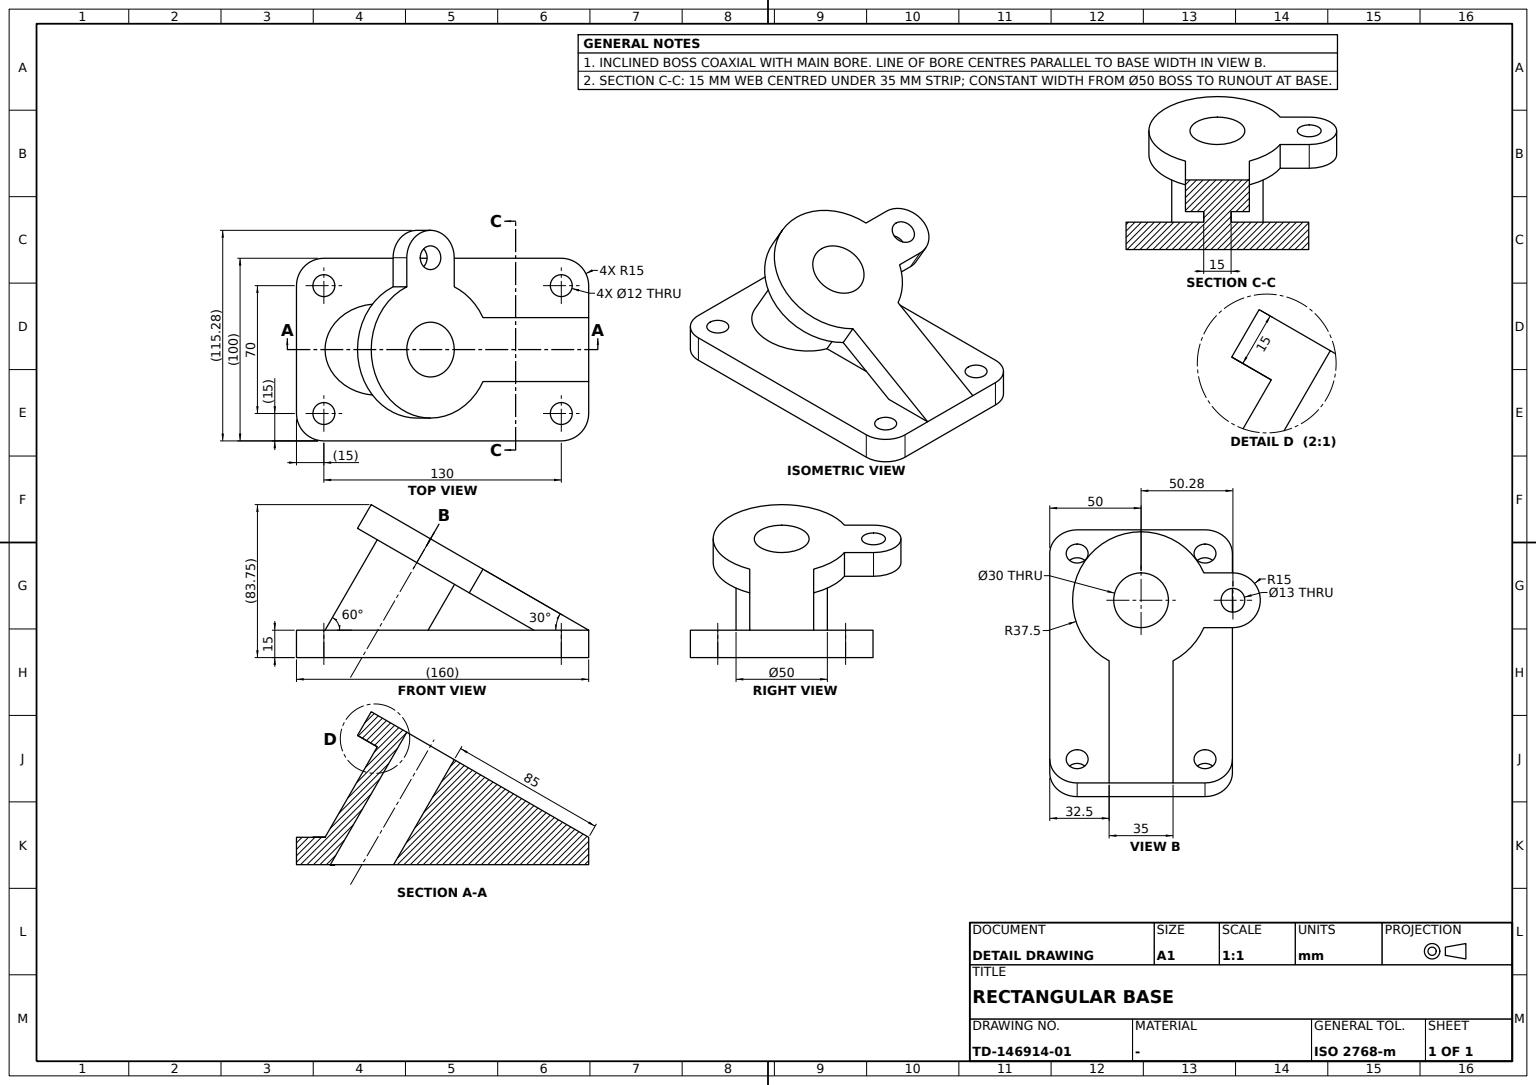
ISO-10303-21;
HEADER;
FILE_DESCRIPTION((''),'2;1');
FILE_NAME('','',(''),(''),'','','');
FILE_SCHEMA(('AUTOMOTIVE_DESIGN'));
ENDSEC;
DATA;
#1=APPLICATION_CONTEXT('');
#2=PRODUCT_CONTEXT('',#1,'mechanical');
#3=PRODUCT('','','',(#2));
#4=PRODUCT_DEFINITION_FORMATION('','',#3);
#5=PRODUCT_DEFINITION_CONTEXT('',#1,'design');
#6=PRODUCT_DEFINITION('','',#4,#5);
#7=PRODUCT_DEFINITION_SHAPE('','',#6);
#8=(LENGTH_UNIT()NAMED_UNIT(*)SI_UNIT(.MILLI.,.METRE.));
#9=(NAMED_UNIT(*)PLANE_ANGLE_UNIT()SI_UNIT($,.RADIAN.));
#10=(NAMED_UNIT(*)SI_UNIT($,.STERADIAN.)SOLID_ANGLE_UNIT());
#11=UNCERTAINTY_MEASURE_WITH_UNIT(LENGTH_MEASURE(0.005),#8,'distance_accuracy_value','');
#12=(GEOMETRIC_REPRESENTATION_CONTEXT(3)GLOBAL_UNCERTAINTY_ASSIGNED_CONTEXT((#11))GLOBAL_UNIT_ASSIGNED_CONTEXT((#8,#9,#10))REPRESENTATION_CONTEXT('',''));
#13=CARTESIAN_POINT('',(-59.,-35.,15.));
#14=VERTEX_POINT('',#13);
#15=CARTESIAN_POINT('',(-71.,-35.,15.));
#16=VERTEX_POINT('',#15);
#17=CARTESIAN_POINT('',(-65.,-35.,15.));
#18=DIRECTION('',(0.,0.,1.));
#19=DIRECTION('',(1.,0.,0.));
#20=AXIS2_PLACEMENT_3D('',#17,#18,#19);
#21=CIRCLE('',#20,6.);
#22=EDGE_CURVE('',#14,#16,#21,.T.);
#23=ORIENTED_EDGE('',*,*,#22,.F.);
#24=EDGE_CURVE('',#16,#14,#21,.T.);
#25=ORIENTED_EDGE('',*,*,#24,.F.);
#26=EDGE_LOOP('',(#23,#25));
#27=FACE_BOUND('',#26,.T.);
#28=CARTESIAN_POINT('',(59.,-35.,15.));
#29=VERTEX_POINT('',#28);
#30=CARTESIAN_POINT('',(71.,-35.,15.));
#31=VERTEX_POINT('',#30);
#32=CARTESIAN_POINT('',(65.,-35.,15.));
#33=AXIS2_PLACEMENT_3D('',#32,#18,#19);
#34=CIRCLE('',#33,6.);
#35=EDGE_CURVE('',#29,#31,#34,.T.);
#36=ORIENTED_EDGE('',*,*,#35,.F.);
#37=EDGE_CURVE('',#31,#29,#34,.T.);
#38=ORIENTED_EDGE('',*,*,#37,.F.);
#39=EDGE_LOOP('',(#36,#38));
#40=FACE_BOUND('',#39,.T.);
#41=CARTESIAN_POINT('',(-71.,35.,15.));
#42=VERTEX_POINT('',#41);
#43=CARTESIAN_POINT('',(-59.,35.,15.));
#44=VERTEX_POINT('',#43);
#45=CARTESIAN_POINT('',(-65.,35.,15.));
#46=AXIS2_PLACEMENT_3D('',#45,#18,#19);
#47=CIRCLE('',#46,6.);
#48=EDGE_CURVE('',#42,#44,#47,.T.);
#49=ORIENTED_EDGE('',*,*,#48,.F.);
#50=EDGE_CURVE('',#44,#42,#47,.T.);
#51=ORIENTED_EDGE('',*,*,#50,.F.);
#52=EDGE_LOOP('',(#49,#51));
#53=FACE_BOUND('',#52,.T.);
#54=CARTESIAN_POINT('',(71.,35.,15.));
#55=VERTEX_POINT('',#54);
#56=CARTESIAN_POINT('',(59.,35.,15.));
#57=VERTEX_POINT('',#56);
#58=CARTESIAN_POINT('',(65.,35.,15.));
#59=AXIS2_PLACEMENT_3D('',#58,#18,#19);
#60=CIRCLE('',#59,6.);
#61=EDGE_CURVE('',#55,#57,#60,.T.);
#62=ORIENTED_EDGE('',*,*,#61,.F.);
#63=EDGE_CURVE('',#57,#55,#60,.T.);
#64=ORIENTED_EDGE('',*,*,#63,.F.);
#65=EDGE_LOOP('',(#62,#64));
#66=FACE_BOUND('',#65,.T.);
#67=CARTESIAN_POINT('',(80.,17.5,15.));
#68=VERTEX_POINT('',#67);
#69=CARTESIAN_POINT('',(80.,35.,15.));
#70=VERTEX_POINT('',#69);
#71=CARTESIAN_POINT('',(80.,-35.,15.));
#72=DIRECTION('',(0.,1.,0.));
#73=VECTOR('',#72,1000.);
#74=LINE('',#71,#73);
#75=EDGE_CURVE('',#68,#70,#74,.T.);
#76=ORIENTED_EDGE('',*,*,#75,.T.);
#77=CARTESIAN_POINT('',(65.,50.,15.));
#78=VERTEX_POINT('',#77);
#79=CIRCLE('',#59,15.);
#80=EDGE_CURVE('',#70,#78,#79,.T.);
#81=ORIENTED_EDGE('',*,*,#80,.T.);
#82=CARTESIAN_POINT('',(-65.,50.,15.));
#83=VERTEX_POINT('',#82);
#84=DIRECTION('',(-1.,0.,0.));
#85=VECTOR('',#84,1000.);
#86=LINE('',#77,#85);
#87=EDGE_CURVE('',#78,#83,#86,.T.);
#88=ORIENTED_EDGE('',*,*,#87,.T.);
#89=CARTESIAN_POINT('',(-80.,35.,15.));
#90=VERTEX_POINT('',#89);
#91=CIRCLE('',#46,15.);
#92=EDGE_CURVE('',#83,#90,#91,.T.);
#93=ORIENTED_EDGE('',*,*,#92,.T.);
#94=CARTESIAN_POINT('',(-80.,-35.,15.));
#95=VERTEX_POINT('',#94);
#96=DIRECTION('',(0.,-1.,0.));
#97=VECTOR('',#96,1000.);
#98=LINE('',#89,#97);
#99=EDGE_CURVE('',#90,#95,#98,.T.);
#100=ORIENTED_EDGE('',*,*,#99,.T.);
#101=CARTESIAN_POINT('',(-65.,-50.,15.));
#102=VERTEX_POINT('',#101);
#103=CIRCLE('',#20,15.);
#104=EDGE_CURVE('',#95,#102,#103,.T.);
#105=ORIENTED_EDGE('',*,*,#104,.T.);
#106=CARTESIAN_POINT('',(65.,-50.,15.));
#107=VERTEX_POINT('',#106);
#108=VECTOR('',#19,1000.);
#109=LINE('',#101,#108);
#110=EDGE_CURVE('',#102,#107,#109,.T.);
#111=ORIENTED_EDGE('',*,*,#110,.T.);
#112=VERTEX_POINT('',#71);
#113=CIRCLE('',#33,15.);
#114=EDGE_CURVE('',#107,#112,#113,.T.);
#115=ORIENTED_EDGE('',*,*,#114,.T.);
#116=CARTESIAN_POINT('',(80.,-17.5,15.));
#117=VERTEX_POINT('',#116);
#118=EDGE_CURVE('',#112,#117,#74,.T.);
#119=ORIENTED_EDGE('',*,*,#118,.T.);
#120=CARTESIAN_POINT('',(50.,-17.5,15.));
#121=VERTEX_POINT('',#120);
#122=CARTESIAN_POINT('',(22.120273,-17.5,15.));
#123=LINE('',#122,#108);
#124=EDGE_CURVE('',#121,#117,#123,.T.);
#125=ORIENTED_EDGE('',*,*,#124,.F.);
#126=CARTESIAN_POINT('',(50.,-7.5,15.));
#127=VERTEX_POINT('',#126);
#128=CARTESIAN_POINT('',(50.,0.,15.));
#129=LINE('',#128,#97);
#130=EDGE_CURVE('',#127,#121,#129,.T.);
#131=ORIENTED_EDGE('',*,*,#130,.F.);
#132=CARTESIAN_POINT('',(-7.932201,-7.5,15.));
#133=VERTEX_POINT('',#132);
#134=CARTESIAN_POINT('',(-65.,-7.5,15.));
#135=LINE('',#134,#85);
#136=EDGE_CURVE('',#127,#133,#135,.T.);
#137=ORIENTED_EDGE('',*,*,#136,.T.);
#138=CARTESIAN_POINT('',(-64.337567,0.,15.));
#139=VERTEX_POINT('',#138);
#140=CARTESIAN_POINT('',(-64.337567,-37.913542,15.));
#141=CARTESIAN_POINT('',(-21.065837,-43.667214,15.));
#142=(BOUNDED_CURVE()B_SPLINE_CURVE(3,(#138,#140,#141,#132),.UNSPECIFIED.,.F.,.F.)B_SPLINE_CURVE_WITH_KNOTS((4,4),(0.,2.8369),.UNSPECIFIED.)CURVE()GEOMETRIC_REPRESENTATION_ITEM()RATIONAL_B_SPLINE_CURVE((1.,0.434505133,0.434505133,1.))REPRESENTATION_ITEM(''));
#143=EDGE_CURVE('',#139,#133,#142,.T.);
#144=ORIENTED_EDGE('',*,*,#143,.F.);
#145=CARTESIAN_POINT('',(-7.932201,7.5,15.));
#146=VERTEX_POINT('',#145);
#147=CARTESIAN_POINT('',(-21.065837,43.667214,15.));
#148=CARTESIAN_POINT('',(-64.337567,37.913542,15.));
#149=(BOUNDED_CURVE()B_SPLINE_CURVE(3,(#145,#147,#148,#138),.UNSPECIFIED.,.F.,.F.)B_SPLINE_CURVE_WITH_KNOTS((4,4),(3.446285308,6.283185307),.UNSPECIFIED.)CURVE()GEOMETRIC_REPRESENTATION_ITEM()RATIONAL_B_SPLINE_CURVE((1.,0.434505133,0.434505133,1.))REPRESENTATION_ITEM(''));
#150=EDGE_CURVE('',#146,#139,#149,.T.);
#151=ORIENTED_EDGE('',*,*,#150,.F.);
#152=CARTESIAN_POINT('',(50.,7.5,15.));
#153=VERTEX_POINT('',#152);
#154=CARTESIAN_POINT('',(-65.,7.5,15.));
#155=LINE('',#154,#108);
#156=EDGE_CURVE('',#146,#153,#155,.T.);
#157=ORIENTED_EDGE('',*,*,#156,.T.);
#158=CARTESIAN_POINT('',(50.,17.5,15.));
#159=VERTEX_POINT('',#158);
#160=EDGE_CURVE('',#159,#153,#129,.T.);
#161=ORIENTED_EDGE('',*,*,#160,.F.);
#162=LINE('',#67,#85);
#163=EDGE_CURVE('',#68,#159,#162,.T.);
#164=ORIENTED_EDGE('',*,*,#163,.F.);
#165=EDGE_LOOP('',(#76,#81,#88,#93,#100,#105,#111,#115,#119,#125,#131,#137,#144,#151,#157,#161,#164));
#166=FACE_BOUND('',#165,.T.);
#167=PLANE('',#20);
#168=ADVANCED_FACE('',(#27,#40,#53,#66,#166),#167,.T.);
#169=CARTESIAN_POINT('',(-35.753175,0.,64.509619));
#170=VERTEX_POINT('',#169);
#171=CARTESIAN_POINT('',(6.550849,7.5,40.085379));
#172=VERTEX_POINT('',#171);
#173=CARTESIAN_POINT('',(-14.10254,0.,52.009619));
#174=DIRECTION('',(-0.5,0.,-0.866025404));
#175=DIRECTION('',(0.866025404,0.,-0.5));
#176=AXIS2_PLACEMENT_3D('',#173,#174,#175);
#177=CIRCLE('',#176,25.);
#178=EDGE_CURVE('',#170,#172,#177,.T.);
#179=ORIENTED_EDGE('',*,*,#178,.F.);
#180=CARTESIAN_POINT('',(6.550849,-7.5,40.085379));
#181=VERTEX_POINT('',#180);
#182=EDGE_CURVE('',#181,#170,#177,.T.);
#183=ORIENTED_EDGE('',*,*,#182,.F.);
#184=CARTESIAN_POINT('',(-14.10254,-7.5,52.009619));
#185=DIRECTION('',(-0.866025404,0.,0.5));
#186=VECTOR('',#185,1000.);
#187=LINE('',#184,#186);
#188=EDGE_CURVE('',#127,#181,#187,.T.);
#189=ORIENTED_EDGE('',*,*,#188,.F.);
#190=ORIENTED_EDGE('',*,*,#130,.T.);
#191=CARTESIAN_POINT('',(14.620273,-17.5,35.426495));
#192=VERTEX_POINT('',#191);
#193=VECTOR('',#175,1000.);
#194=LINE('',#191,#193);
#195=EDGE_CURVE('',#192,#121,#194,.T.);
#196=ORIENTED_EDGE('',*,*,#195,.F.);
#197=CARTESIAN_POINT('',(-46.578493,0.,70.759619));
#198=VERTEX_POINT('',#197);
#199=DIRECTION('',(0.5,0.,0.866025404));
#200=AXIS2_PLACEMENT_3D('',#173,#199,#175);
#201=CIRCLE('',#200,37.5);
#202=EDGE_CURVE('',#198,#192,#201,.T.);
#203=ORIENTED_EDGE('',*,*,#202,.F.);
#204=CARTESIAN_POINT('',(-27.092921,34.369318,59.509619));
#205=VERTEX_POINT('',#204);
#206=EDGE_CURVE('',#205,#198,#201,.T.);
#207=ORIENTED_EDGE('',*,*,#206,.F.);
#208=CARTESIAN_POINT('',(-27.092921,50.281547,59.509619));
#209=VERTEX_POINT('',#208);
#210=LINE('',#208,#97);
#211=EDGE_CURVE('',#209,#205,#210,.T.);
#212=ORIENTED_EDGE('',*,*,#211,.F.);
#213=CARTESIAN_POINT('',(-1.112159,50.281547,44.509619));
#214=VERTEX_POINT('',#213);
#215=CARTESIAN_POINT('',(-14.10254,50.281547,52.009619));
#216=AXIS2_PLACEMENT_3D('',#215,#199,#175);
#217=CIRCLE('',#216,15.);
#218=EDGE_CURVE('',#214,#209,#217,.T.);
#219=ORIENTED_EDGE('',*,*,#218,.F.);
#220=CARTESIAN_POINT('',(-1.112159,34.369318,44.509619));
#221=VERTEX_POINT('',#220);
#222=LINE('',#220,#73);
#223=EDGE_CURVE('',#221,#214,#222,.T.);
#224=ORIENTED_EDGE('',*,*,#223,.F.);
#225=CARTESIAN_POINT('',(14.620273,17.5,35.426495));
#226=VERTEX_POINT('',#225);
#227=EDGE_CURVE('',#226,#221,#201,.T.);
#228=ORIENTED_EDGE('',*,*,#227,.F.);
#229=CARTESIAN_POINT('',(72.5,17.5,2.009619));
#230=LINE('',#229,#186);
#231=EDGE_CURVE('',#159,#226,#230,.T.);
#232=ORIENTED_EDGE('',*,*,#231,.F.);
#233=ORIENTED_EDGE('',*,*,#160,.T.);
#234=CARTESIAN_POINT('',(-14.10254,7.5,52.009619));
#235=LINE('',#234,#193);
#236=EDGE_CURVE('',#172,#153,#235,.T.);
#237=ORIENTED_EDGE('',*,*,#236,.F.);
#238=EDGE_LOOP('',(#179,#183,#189,#190,#196,#203,#207,#212,#219,#224,#228,#232,#233,#237));
#239=FACE_BOUND('',#238,.T.);
#240=CARTESIAN_POINT('',(-19.731706,50.281547,55.259619));
#241=VERTEX_POINT('',#240);
#242=CARTESIAN_POINT('',(-8.473375,50.281547,48.759619));
#243=VERTEX_POINT('',#242);
#244=CIRCLE('',#216,6.5);
#245=EDGE_CURVE('',#241,#243,#244,.T.);
#246=ORIENTED_EDGE('',*,*,#245,.T.);
#247=EDGE_CURVE('',#243,#241,#244,.T.);
#248=ORIENTED_EDGE('',*,*,#247,.T.);
#249=EDGE_LOOP('',(#246,#248));
#250=FACE_BOUND('',#249,.T.);
#251=PLANE('',#200);
#252=ADVANCED_FACE('',(#239,#250),#251,.F.);
#253=CARTESIAN_POINT('',(6.387841,0.,57.5));
#254=VERTEX_POINT('',#253);
#255=CARTESIAN_POINT('',(-19.592921,0.,72.5));
#256=VERTEX_POINT('',#255);
#257=CARTESIAN_POINT('',(-6.60254,0.,65.));
#258=AXIS2_PLACEMENT_3D('',#257,#199,#72);
#259=CIRCLE('',#258,15.);
#260=EDGE_CURVE('',#254,#256,#259,.T.);
#261=ORIENTED_EDGE('',*,*,#260,.F.);
#262=EDGE_CURVE('',#256,#254,#259,.T.);
#263=ORIENTED_EDGE('',*,*,#262,.F.);
#264=EDGE_LOOP('',(#261,#263));
#265=FACE_BOUND('',#264,.T.);
#266=CARTESIAN_POINT('',(-19.592921,34.369318,72.5));
#267=VERTEX_POINT('',#266);
#268=CARTESIAN_POINT('',(-39.078493,0.,83.75));
#269=VERTEX_POINT('',#268);
#270=AXIS2_PLACEMENT_3D('',#257,#199,#175);
#271=CIRCLE('',#270,37.5);
#272=EDGE_CURVE('',#267,#269,#271,.T.);
#273=ORIENTED_EDGE('',*,*,#272,.T.);
#274=CARTESIAN_POINT('',(22.120273,-17.5,48.416876));
#275=VERTEX_POINT('',#274);
#276=EDGE_CURVE('',#269,#275,#271,.T.);
#277=ORIENTED_EDGE('',*,*,#276,.T.);
#278=LINE('',#274,#193);
#279=EDGE_CURVE('',#275,#117,#278,.T.);
#280=ORIENTED_EDGE('',*,*,#279,.T.);
#281=LINE('',#116,#73);
#282=EDGE_CURVE('',#117,#68,#281,.T.);
#283=ORIENTED_EDGE('',*,*,#282,.T.);
#284=CARTESIAN_POINT('',(22.120273,17.5,48.416876));
#285=VERTEX_POINT('',#284);
#286=LINE('',#67,#186);
#287=EDGE_CURVE('',#68,#285,#286,.T.);
#288=ORIENTED_EDGE('',*,*,#287,.T.);
#289=CARTESIAN_POINT('',(6.387841,34.369318,57.5));
#290=VERTEX_POINT('',#289);
#291=EDGE_CURVE('',#285,#290,#271,.T.);
#292=ORIENTED_EDGE('',*,*,#291,.T.);
#293=CARTESIAN_POINT('',(6.387841,50.281547,57.5));
#294=VERTEX_POINT('',#293);
#295=LINE('',#289,#73);
#296=EDGE_CURVE('',#290,#294,#295,.T.);
#297=ORIENTED_EDGE('',*,*,#296,.T.);
#298=CARTESIAN_POINT('',(-19.592921,50.281547,72.5));
#299=VERTEX_POINT('',#298);
#300=CARTESIAN_POINT('',(-6.60254,50.281547,65.));
#301=AXIS2_PLACEMENT_3D('',#300,#199,#175);
#302=CIRCLE('',#301,15.);
#303=EDGE_CURVE('',#294,#299,#302,.T.);
#304=ORIENTED_EDGE('',*,*,#303,.T.);
#305=LINE('',#298,#97);
#306=EDGE_CURVE('',#299,#267,#305,.T.);
#307=ORIENTED_EDGE('',*,*,#306,.T.);
#308=EDGE_LOOP('',(#273,#277,#280,#283,#288,#292,#297,#304,#307));
#309=FACE_BOUND('',#308,.T.);
#310=CARTESIAN_POINT('',(-12.231706,50.281547,68.25));
#311=VERTEX_POINT('',#310);
#312=CARTESIAN_POINT('',(-0.973375,50.281547,61.75));
#313=VERTEX_POINT('',#312);
#314=CIRCLE('',#301,6.5);
#315=EDGE_CURVE('',#311,#313,#314,.T.);
#316=ORIENTED_EDGE('',*,*,#315,.F.);
#317=EDGE_CURVE('',#313,#311,#314,.T.);
#318=ORIENTED_EDGE('',*,*,#317,.F.);
#319=EDGE_LOOP('',(#316,#318));
#320=FACE_BOUND('',#319,.T.);
#321=PLANE('',#270);
#322=ADVANCED_FACE('',(#265,#309,#320),#321,.T.);
#323=ORIENTED_EDGE('',*,*,#245,.F.);
#324=VECTOR('',#174,1000.);
#325=LINE('',#310,#324);
#326=EDGE_CURVE('',#241,#311,#325,.F.);
#327=ORIENTED_EDGE('',*,*,#326,.T.);
#328=ORIENTED_EDGE('',*,*,#315,.T.);
#329=LINE('',#312,#324);
#330=EDGE_CURVE('',#313,#243,#329,.T.);
#331=ORIENTED_EDGE('',*,*,#330,.T.);
#332=EDGE_LOOP('',(#323,#327,#328,#331));
#333=FACE_BOUND('',#332,.T.);
#334=AXIS2_PLACEMENT_3D('',#300,#174,#185);
#335=CYLINDRICAL_SURFACE('',#334,6.5);
#336=ADVANCED_FACE('',(#333),#335,.F.);
#337=ORIENTED_EDGE('',*,*,#143,.T.);
#338=CARTESIAN_POINT('',(14.050849,-7.5,53.07576));
#339=LINE('',#338,#324);
#340=EDGE_CURVE('',#181,#133,#339,.T.);
#341=ORIENTED_EDGE('',*,*,#340,.F.);
#342=ORIENTED_EDGE('',*,*,#182,.T.);
#343=CARTESIAN_POINT('',(-28.253175,0.,77.5));
#344=LINE('',#343,#324);
#345=EDGE_CURVE('',#170,#139,#344,.T.);
#346=ORIENTED_EDGE('',*,*,#345,.T.);
#347=EDGE_LOOP('',(#337,#341,#342,#346));
#348=FACE_BOUND('',#347,.T.);
#349=AXIS2_PLACEMENT_3D('',#257,#174,#185);
#350=CYLINDRICAL_SURFACE('',#349,25.);
#351=ADVANCED_FACE('',(#348),#350,.T.);
#352=LINE('',#268,#324);
#353=EDGE_CURVE('',#269,#198,#352,.T.);
#354=ORIENTED_EDGE('',*,*,#353,.F.);
#355=ORIENTED_EDGE('',*,*,#272,.F.);
#356=LINE('',#266,#324);
#357=EDGE_CURVE('',#267,#205,#356,.T.);
#358=ORIENTED_EDGE('',*,*,#357,.T.);
#359=ORIENTED_EDGE('',*,*,#206,.T.);
#360=EDGE_LOOP('',(#354,#355,#358,#359));
#361=FACE_BOUND('',#360,.T.);
#362=CYLINDRICAL_SURFACE('',#349,37.5);
#363=ADVANCED_FACE('',(#361),#362,.T.);
#364=ORIENTED_EDGE('',*,*,#75,.F.);
#365=ORIENTED_EDGE('',*,*,#282,.F.);
#366=ORIENTED_EDGE('',*,*,#118,.F.);
#367=CARTESIAN_POINT('',(80.,-35.,0.));
#368=VERTEX_POINT('',#367);
#369=DIRECTION('',(0.,0.,-1.));
#370=VECTOR('',#369,1000.);
#371=LINE('',#71,#370);
#372=EDGE_CURVE('',#112,#368,#371,.T.);
#373=ORIENTED_EDGE('',*,*,#372,.T.);
#374=CARTESIAN_POINT('',(80.,35.,0.));
#375=VERTEX_POINT('',#374);
#376=LINE('',#367,#73);
#377=EDGE_CURVE('',#368,#375,#376,.T.);
#378=ORIENTED_EDGE('',*,*,#377,.T.);
#379=LINE('',#69,#370);
#380=EDGE_CURVE('',#70,#375,#379,.T.);
#381=ORIENTED_EDGE('',*,*,#380,.F.);
#382=EDGE_LOOP('',(#364,#365,#366,#373,#378,#381));
#383=FACE_BOUND('',#382,.T.);
#384=AXIS2_PLACEMENT_3D('',#71,#84,#18);
#385=PLANE('',#384);
#386=ADVANCED_FACE('',(#383),#385,.F.);
#387=ORIENTED_EDGE('',*,*,#353,.T.);
#388=ORIENTED_EDGE('',*,*,#202,.T.);
#389=LINE('',#274,#324);
#390=EDGE_CURVE('',#275,#192,#389,.T.);
#391=ORIENTED_EDGE('',*,*,#390,.F.);
#392=ORIENTED_EDGE('',*,*,#276,.F.);
#393=EDGE_LOOP('',(#387,#388,#391,#392));
#394=FACE_BOUND('',#393,.T.);
#395=ADVANCED_FACE('',(#394),#362,.T.);
#396=ORIENTED_EDGE('',*,*,#306,.F.);
#397=LINE('',#298,#324);
#398=EDGE_CURVE('',#299,#209,#397,.T.);
#399=ORIENTED_EDGE('',*,*,#398,.T.);
#400=ORIENTED_EDGE('',*,*,#211,.T.);
#401=ORIENTED_EDGE('',*,*,#357,.F.);
#402=EDGE_LOOP('',(#396,#399,#400,#401));
#403=FACE_BOUND('',#402,.T.);
#404=AXIS2_PLACEMENT_3D('',#298,#175,#174);
#405=PLANE('',#404);
#406=ADVANCED_FACE('',(#403),#405,.F.);
#407=CARTESIAN_POINT('',(-65.,50.,0.));
#408=VERTEX_POINT('',#407);
#409=CARTESIAN_POINT('',(-80.,35.,0.));
#410=VERTEX_POINT('',#409);
#411=CARTESIAN_POINT('',(-65.,35.,0.));
#412=AXIS2_PLACEMENT_3D('',#411,#18,#19);
#413=CIRCLE('',#412,15.);
#414=EDGE_CURVE('',#408,#410,#413,.T.);
#415=ORIENTED_EDGE('',*,*,#414,.F.);
#416=CARTESIAN_POINT('',(65.,50.,0.));
#417=VERTEX_POINT('',#416);
#418=LINE('',#416,#85);
#419=EDGE_CURVE('',#417,#408,#418,.T.);
#420=ORIENTED_EDGE('',*,*,#419,.F.);
#421=CARTESIAN_POINT('',(65.,35.,0.));
#422=AXIS2_PLACEMENT_3D('',#421,#18,#19);
#423=CIRCLE('',#422,15.);
#424=EDGE_CURVE('',#375,#417,#423,.T.);
#425=ORIENTED_EDGE('',*,*,#424,.F.);
#426=ORIENTED_EDGE('',*,*,#377,.F.);
#427=CARTESIAN_POINT('',(65.,-50.,0.));
#428=VERTEX_POINT('',#427);
#429=CARTESIAN_POINT('',(65.,-35.,0.));
#430=AXIS2_PLACEMENT_3D('',#429,#18,#19);
#431=CIRCLE('',#430,15.);
#432=EDGE_CURVE('',#428,#368,#431,.T.);
#433=ORIENTED_EDGE('',*,*,#432,.F.);
#434=CARTESIAN_POINT('',(-65.,-50.,0.));
#435=VERTEX_POINT('',#434);
#436=LINE('',#434,#108);
#437=EDGE_CURVE('',#435,#428,#436,.T.);
#438=ORIENTED_EDGE('',*,*,#437,.F.);
#439=CARTESIAN_POINT('',(-80.,-35.,0.));
#440=VERTEX_POINT('',#439);
#441=CARTESIAN_POINT('',(-65.,-35.,0.));
#442=AXIS2_PLACEMENT_3D('',#441,#18,#19);
#443=CIRCLE('',#442,15.);
#444=EDGE_CURVE('',#440,#435,#443,.T.);
#445=ORIENTED_EDGE('',*,*,#444,.F.);
#446=LINE('',#409,#97);
#447=EDGE_CURVE('',#410,#440,#446,.T.);
#448=ORIENTED_EDGE('',*,*,#447,.F.);
#449=EDGE_LOOP('',(#415,#420,#425,#426,#433,#438,#445,#448));
#450=FACE_BOUND('',#449,.T.);
#451=CARTESIAN_POINT('',(-71.,35.,0.));
#452=VERTEX_POINT('',#451);
#453=CARTESIAN_POINT('',(-59.,35.,0.));
#454=VERTEX_POINT('',#453);
#455=CIRCLE('',#412,6.);
#456=EDGE_CURVE('',#452,#454,#455,.T.);
#457=ORIENTED_EDGE('',*,*,#456,.T.);
#458=EDGE_CURVE('',#454,#452,#455,.T.);
#459=ORIENTED_EDGE('',*,*,#458,.T.);
#460=EDGE_LOOP('',(#457,#459));
#461=FACE_BOUND('',#460,.T.);
#462=CARTESIAN_POINT('',(71.,35.,0.));
#463=VERTEX_POINT('',#462);
#464=CARTESIAN_POINT('',(59.,35.,0.));
#465=VERTEX_POINT('',#464);
#466=CIRCLE('',#422,6.);
#467=EDGE_CURVE('',#463,#465,#466,.T.);
#468=ORIENTED_EDGE('',*,*,#467,.T.);
#469=EDGE_CURVE('',#465,#463,#466,.T.);
#470=ORIENTED_EDGE('',*,*,#469,.T.);
#471=EDGE_LOOP('',(#468,#470));
#472=FACE_BOUND('',#471,.T.);
#473=CARTESIAN_POINT('',(59.,-35.,0.));
#474=VERTEX_POINT('',#473);
#475=CARTESIAN_POINT('',(71.,-35.,0.));
#476=VERTEX_POINT('',#475);
#477=CIRCLE('',#430,6.);
#478=EDGE_CURVE('',#474,#476,#477,.T.);
#479=ORIENTED_EDGE('',*,*,#478,.T.);
#480=EDGE_CURVE('',#476,#474,#477,.T.);
#481=ORIENTED_EDGE('',*,*,#480,.T.);
#482=EDGE_LOOP('',(#479,#481));
#483=FACE_BOUND('',#482,.T.);
#484=CARTESIAN_POINT('',(-61.450816,0.,0.));
#485=VERTEX_POINT('',#484);
#486=CARTESIAN_POINT('',(-26.8098,0.,0.));
#487=VERTEX_POINT('',#486);
#488=CARTESIAN_POINT('',(-61.450816,30.,0.));
#489=CARTESIAN_POINT('',(-26.8098,30.,0.));
#490=(BOUNDED_CURVE()B_SPLINE_CURVE(3,(#484,#488,#489,#486),.UNSPECIFIED.,.F.,.F.)B_SPLINE_CURVE_WITH_KNOTS((4,4),(0.,3.141592654),.UNSPECIFIED.)CURVE()GEOMETRIC_REPRESENTATION_ITEM()RATIONAL_B_SPLINE_CURVE((1.,0.333333333,0.333333333,1.))REPRESENTATION_ITEM(''));
#491=EDGE_CURVE('',#485,#487,#490,.T.);
#492=ORIENTED_EDGE('',*,*,#491,.F.);
#493=CARTESIAN_POINT('',(-26.8098,-30.,0.));
#494=CARTESIAN_POINT('',(-61.450816,-30.,0.));
#495=(BOUNDED_CURVE()B_SPLINE_CURVE(3,(#486,#493,#494,#484),.UNSPECIFIED.,.F.,.F.)B_SPLINE_CURVE_WITH_KNOTS((4,4),(3.141592654,6.283185307),.UNSPECIFIED.)CURVE()GEOMETRIC_REPRESENTATION_ITEM()RATIONAL_B_SPLINE_CURVE((1.,0.333333333,0.333333333,1.))REPRESENTATION_ITEM(''));
#496=EDGE_CURVE('',#487,#485,#495,.T.);
#497=ORIENTED_EDGE('',*,*,#496,.F.);
#498=EDGE_LOOP('',(#492,#497));
#499=FACE_BOUND('',#498,.T.);
#500=CARTESIAN_POINT('',(-71.,-35.,0.));
#501=VERTEX_POINT('',#500);
#502=CARTESIAN_POINT('',(-59.,-35.,0.));
#503=VERTEX_POINT('',#502);
#504=CIRCLE('',#442,6.);
#505=EDGE_CURVE('',#501,#503,#504,.T.);
#506=ORIENTED_EDGE('',*,*,#505,.T.);
#507=EDGE_CURVE('',#503,#501,#504,.T.);
#508=ORIENTED_EDGE('',*,*,#507,.T.);
#509=EDGE_LOOP('',(#506,#508));
#510=FACE_BOUND('',#509,.T.);
#511=PLANE('',#442);
#512=ADVANCED_FACE('',(#450,#461,#472,#483,#499,#510),#511,.F.);
#513=ORIENTED_EDGE('',*,*,#156,.F.);
#514=CARTESIAN_POINT('',(14.050849,7.5,53.07576));
#515=VECTOR('',#199,1000.);
#516=LINE('',#514,#515);
#517=EDGE_CURVE('',#146,#172,#516,.T.);
#518=ORIENTED_EDGE('',*,*,#517,.T.);
#519=ORIENTED_EDGE('',*,*,#236,.T.);
#520=EDGE_LOOP('',(#513,#518,#519));
#521=FACE_BOUND('',#520,.T.);
#522=CARTESIAN_POINT('',(86.495191,7.5,11.25));
#523=AXIS2_PLACEMENT_3D('',#522,#96,#369);
#524=PLANE('',#523);
#525=ADVANCED_FACE('',(#521),#524,.F.);
#526=LINE('',#15,#370);
#527=EDGE_CURVE('',#501,#16,#526,.F.);
#528=ORIENTED_EDGE('',*,*,#527,.F.);
#529=ORIENTED_EDGE('',*,*,#507,.F.);
#530=LINE('',#13,#370);
#531=EDGE_CURVE('',#14,#503,#530,.T.);
#532=ORIENTED_EDGE('',*,*,#531,.F.);
#533=ORIENTED_EDGE('',*,*,#22,.T.);
#534=EDGE_LOOP('',(#528,#529,#532,#533));
#535=FACE_BOUND('',#534,.T.);
#536=AXIS2_PLACEMENT_3D('',#17,#369,#84);
#537=CYLINDRICAL_SURFACE('',#536,6.);
#538=ADVANCED_FACE('',(#535),#537,.F.);
#539=ORIENTED_EDGE('',*,*,#345,.F.);
#540=ORIENTED_EDGE('',*,*,#178,.T.);
#541=ORIENTED_EDGE('',*,*,#517,.F.);
#542=ORIENTED_EDGE('',*,*,#150,.T.);
#543=EDGE_LOOP('',(#539,#540,#541,#542));
#544=FACE_BOUND('',#543,.T.);
#545=ADVANCED_FACE('',(#544),#350,.T.);
#546=ORIENTED_EDGE('',*,*,#99,.F.);
#547=LINE('',#89,#370);
#548=EDGE_CURVE('',#90,#410,#547,.T.);
#549=ORIENTED_EDGE('',*,*,#548,.T.);
#550=ORIENTED_EDGE('',*,*,#447,.T.);
#551=LINE('',#94,#370);
#552=EDGE_CURVE('',#95,#440,#551,.T.);
#553=ORIENTED_EDGE('',*,*,#552,.F.);
#554=EDGE_LOOP('',(#546,#549,#550,#553));
#555=FACE_BOUND('',#554,.T.);
#556=AXIS2_PLACEMENT_3D('',#89,#19,#369);
#557=PLANE('',#556);
#558=ADVANCED_FACE('',(#555),#557,.F.);
#559=ORIENTED_EDGE('',*,*,#432,.T.);
#560=ORIENTED_EDGE('',*,*,#372,.F.);
#561=ORIENTED_EDGE('',*,*,#114,.F.);
#562=LINE('',#106,#370);
#563=EDGE_CURVE('',#107,#428,#562,.T.);
#564=ORIENTED_EDGE('',*,*,#563,.T.);
#565=EDGE_LOOP('',(#559,#560,#561,#564));
#566=FACE_BOUND('',#565,.T.);
#567=AXIS2_PLACEMENT_3D('',#32,#369,#84);
#568=CYLINDRICAL_SURFACE('',#567,15.);
#569=ADVANCED_FACE('',(#566),#568,.T.);
#570=ORIENTED_EDGE('',*,*,#552,.T.);
#571=ORIENTED_EDGE('',*,*,#444,.T.);
#572=LINE('',#101,#370);
#573=EDGE_CURVE('',#102,#435,#572,.T.);
#574=ORIENTED_EDGE('',*,*,#573,.F.);
#575=ORIENTED_EDGE('',*,*,#104,.F.);
#576=EDGE_LOOP('',(#570,#571,#574,#575));
#577=FACE_BOUND('',#576,.T.);
#578=CYLINDRICAL_SURFACE('',#536,15.);
#579=ADVANCED_FACE('',(#577),#578,.T.);
#580=ORIENTED_EDGE('',*,*,#260,.T.);
#581=LINE('',#255,#324);
#582=EDGE_CURVE('',#256,#485,#581,.T.);
#583=ORIENTED_EDGE('',*,*,#582,.T.);
#584=ORIENTED_EDGE('',*,*,#491,.T.);
#585=LINE('',#253,#324);
#586=EDGE_CURVE('',#487,#254,#585,.F.);
#587=ORIENTED_EDGE('',*,*,#586,.T.);
#588=EDGE_LOOP('',(#580,#583,#584,#587));
#589=FACE_BOUND('',#588,.T.);
#590=CYLINDRICAL_SURFACE('',#349,15.);
#591=ADVANCED_FACE('',(#589),#590,.F.);
#592=ORIENTED_EDGE('',*,*,#92,.F.);
#593=LINE('',#82,#370);
#594=EDGE_CURVE('',#83,#408,#593,.T.);
#595=ORIENTED_EDGE('',*,*,#594,.T.);
#596=ORIENTED_EDGE('',*,*,#414,.T.);
#597=ORIENTED_EDGE('',*,*,#548,.F.);
#598=EDGE_LOOP('',(#592,#595,#596,#597));
#599=FACE_BOUND('',#598,.T.);
#600=AXIS2_PLACEMENT_3D('',#45,#369,#84);
#601=CYLINDRICAL_SURFACE('',#600,15.);
#602=ADVANCED_FACE('',(#599),#601,.T.);
#603=ORIENTED_EDGE('',*,*,#287,.F.);
#604=ORIENTED_EDGE('',*,*,#163,.T.);
#605=ORIENTED_EDGE('',*,*,#231,.T.);
#606=LINE('',#284,#324);
#607=EDGE_CURVE('',#285,#226,#606,.T.);
#608=ORIENTED_EDGE('',*,*,#607,.F.);
#609=EDGE_LOOP('',(#603,#604,#605,#608));
#610=FACE_BOUND('',#609,.T.);
#611=AXIS2_PLACEMENT_3D('',#67,#96,#369);
#612=PLANE('',#611);
#613=ADVANCED_FACE('',(#610),#612,.F.);
#614=ORIENTED_EDGE('',*,*,#527,.T.);
#615=ORIENTED_EDGE('',*,*,#24,.T.);
#616=ORIENTED_EDGE('',*,*,#531,.T.);
#617=ORIENTED_EDGE('',*,*,#505,.F.);
#618=EDGE_LOOP('',(#614,#615,#616,#617));
#619=FACE_BOUND('',#618,.T.);
#620=ADVANCED_FACE('',(#619),#537,.F.);
#621=LINE('',#30,#370);
#622=EDGE_CURVE('',#476,#31,#621,.F.);
#623=ORIENTED_EDGE('',*,*,#622,.F.);
#624=ORIENTED_EDGE('',*,*,#478,.F.);
#625=LINE('',#28,#370);
#626=EDGE_CURVE('',#29,#474,#625,.T.);
#627=ORIENTED_EDGE('',*,*,#626,.F.);
#628=ORIENTED_EDGE('',*,*,#35,.T.);
#629=EDGE_LOOP('',(#623,#624,#627,#628));
#630=FACE_BOUND('',#629,.T.);
#631=CYLINDRICAL_SURFACE('',#567,6.);
#632=ADVANCED_FACE('',(#630),#631,.F.);
#633=ORIENTED_EDGE('',*,*,#469,.F.);
#634=LINE('',#56,#370);
#635=EDGE_CURVE('',#465,#57,#634,.F.);
#636=ORIENTED_EDGE('',*,*,#635,.T.);
#637=ORIENTED_EDGE('',*,*,#63,.T.);
#638=LINE('',#54,#370);
#639=EDGE_CURVE('',#55,#463,#638,.T.);
#640=ORIENTED_EDGE('',*,*,#639,.T.);
#641=EDGE_LOOP('',(#633,#636,#637,#640));
#642=FACE_BOUND('',#641,.T.);
#643=AXIS2_PLACEMENT_3D('',#58,#369,#84);
#644=CYLINDRICAL_SURFACE('',#643,6.);
#645=ADVANCED_FACE('',(#642),#644,.F.);
#646=ORIENTED_EDGE('',*,*,#296,.F.);
#647=LINE('',#289,#324);
#648=EDGE_CURVE('',#290,#221,#647,.T.);
#649=ORIENTED_EDGE('',*,*,#648,.T.);
#650=ORIENTED_EDGE('',*,*,#223,.T.);
#651=LINE('',#293,#324);
#652=EDGE_CURVE('',#294,#214,#651,.T.);
#653=ORIENTED_EDGE('',*,*,#652,.F.);
#654=EDGE_LOOP('',(#646,#649,#650,#653));
#655=FACE_BOUND('',#654,.T.);
#656=AXIS2_PLACEMENT_3D('',#289,#185,#199);
#657=PLANE('',#656);
#658=ADVANCED_FACE('',(#655),#657,.F.);
#659=ORIENTED_EDGE('',*,*,#639,.F.);
#660=ORIENTED_EDGE('',*,*,#61,.T.);
#661=ORIENTED_EDGE('',*,*,#635,.F.);
#662=ORIENTED_EDGE('',*,*,#467,.F.);
#663=EDGE_LOOP('',(#659,#660,#661,#662));
#664=FACE_BOUND('',#663,.T.);
#665=ADVANCED_FACE('',(#664),#644,.F.);
#666=ORIENTED_EDGE('',*,*,#247,.F.);
#667=ORIENTED_EDGE('',*,*,#330,.F.);
#668=ORIENTED_EDGE('',*,*,#317,.T.);
#669=ORIENTED_EDGE('',*,*,#326,.F.);
#670=EDGE_LOOP('',(#666,#667,#668,#669));
#671=FACE_BOUND('',#670,.T.);
#672=ADVANCED_FACE('',(#671),#335,.F.);
#673=ORIENTED_EDGE('',*,*,#80,.F.);
#674=ORIENTED_EDGE('',*,*,#380,.T.);
#675=ORIENTED_EDGE('',*,*,#424,.T.);
#676=LINE('',#77,#370);
#677=EDGE_CURVE('',#78,#417,#676,.T.);
#678=ORIENTED_EDGE('',*,*,#677,.F.);
#679=EDGE_LOOP('',(#673,#674,#675,#678));
#680=FACE_BOUND('',#679,.T.);
#681=CYLINDRICAL_SURFACE('',#643,15.);
#682=ADVANCED_FACE('',(#680),#681,.T.);
#683=ORIENTED_EDGE('',*,*,#594,.F.);
#684=ORIENTED_EDGE('',*,*,#87,.F.);
#685=ORIENTED_EDGE('',*,*,#677,.T.);
#686=ORIENTED_EDGE('',*,*,#419,.T.);
#687=EDGE_LOOP('',(#683,#684,#685,#686));
#688=FACE_BOUND('',#687,.T.);
#689=AXIS2_PLACEMENT_3D('',#77,#96,#369);
#690=PLANE('',#689);
#691=ADVANCED_FACE('',(#688),#690,.F.);
#692=ORIENTED_EDGE('',*,*,#398,.F.);
#693=ORIENTED_EDGE('',*,*,#303,.F.);
#694=ORIENTED_EDGE('',*,*,#652,.T.);
#695=ORIENTED_EDGE('',*,*,#218,.T.);
#696=EDGE_LOOP('',(#692,#693,#694,#695));
#697=FACE_BOUND('',#696,.T.);
#698=CYLINDRICAL_SURFACE('',#334,15.);
#699=ADVANCED_FACE('',(#697),#698,.T.);
#700=ORIENTED_EDGE('',*,*,#622,.T.);
#701=ORIENTED_EDGE('',*,*,#37,.T.);
#702=ORIENTED_EDGE('',*,*,#626,.T.);
#703=ORIENTED_EDGE('',*,*,#480,.F.);
#704=EDGE_LOOP('',(#700,#701,#702,#703));
#705=FACE_BOUND('',#704,.T.);
#706=ADVANCED_FACE('',(#705),#631,.F.);
#707=LINE('',#41,#370);
#708=EDGE_CURVE('',#452,#42,#707,.F.);
#709=ORIENTED_EDGE('',*,*,#708,.T.);
#710=ORIENTED_EDGE('',*,*,#48,.T.);
#711=LINE('',#43,#370);
#712=EDGE_CURVE('',#44,#454,#711,.T.);
#713=ORIENTED_EDGE('',*,*,#712,.T.);
#714=ORIENTED_EDGE('',*,*,#456,.F.);
#715=EDGE_LOOP('',(#709,#710,#713,#714));
#716=FACE_BOUND('',#715,.T.);
#717=CYLINDRICAL_SURFACE('',#600,6.);
#718=ADVANCED_FACE('',(#716),#717,.F.);
#719=ORIENTED_EDGE('',*,*,#227,.T.);
#720=ORIENTED_EDGE('',*,*,#648,.F.);
#721=ORIENTED_EDGE('',*,*,#291,.F.);
#722=ORIENTED_EDGE('',*,*,#607,.T.);
#723=EDGE_LOOP('',(#719,#720,#721,#722));
#724=FACE_BOUND('',#723,.T.);
#725=ADVANCED_FACE('',(#724),#362,.T.);
#726=ORIENTED_EDGE('',*,*,#712,.F.);
#727=ORIENTED_EDGE('',*,*,#50,.T.);
#728=ORIENTED_EDGE('',*,*,#708,.F.);
#729=ORIENTED_EDGE('',*,*,#458,.F.);
#730=EDGE_LOOP('',(#726,#727,#728,#729));
#731=FACE_BOUND('',#730,.T.);
#732=ADVANCED_FACE('',(#731),#717,.F.);
#733=ORIENTED_EDGE('',*,*,#586,.F.);
#734=ORIENTED_EDGE('',*,*,#496,.T.);
#735=ORIENTED_EDGE('',*,*,#582,.F.);
#736=ORIENTED_EDGE('',*,*,#262,.T.);
#737=EDGE_LOOP('',(#733,#734,#735,#736));
#738=FACE_BOUND('',#737,.T.);
#739=ADVANCED_FACE('',(#738),#590,.F.);
#740=ORIENTED_EDGE('',*,*,#110,.F.);
#741=ORIENTED_EDGE('',*,*,#573,.T.);
#742=ORIENTED_EDGE('',*,*,#437,.T.);
#743=ORIENTED_EDGE('',*,*,#563,.F.);
#744=EDGE_LOOP('',(#740,#741,#742,#743));
#745=FACE_BOUND('',#744,.T.);
#746=AXIS2_PLACEMENT_3D('',#101,#72,#18);
#747=PLANE('',#746);
#748=ADVANCED_FACE('',(#745),#747,.F.);
#749=ORIENTED_EDGE('',*,*,#390,.T.);
#750=ORIENTED_EDGE('',*,*,#195,.T.);
#751=ORIENTED_EDGE('',*,*,#124,.T.);
#752=ORIENTED_EDGE('',*,*,#279,.F.);
#753=EDGE_LOOP('',(#749,#750,#751,#752));
#754=FACE_BOUND('',#753,.T.);
#755=AXIS2_PLACEMENT_3D('',#274,#72,#18);
#756=PLANE('',#755);
#757=ADVANCED_FACE('',(#754),#756,.F.);
#758=ORIENTED_EDGE('',*,*,#188,.T.);
#759=ORIENTED_EDGE('',*,*,#340,.T.);
#760=ORIENTED_EDGE('',*,*,#136,.F.);
#761=EDGE_LOOP('',(#758,#759,#760));
#762=FACE_BOUND('',#761,.T.);
#763=CARTESIAN_POINT('',(6.387841,-7.5,57.5));
#764=AXIS2_PLACEMENT_3D('',#763,#72,#18);
#765=PLANE('',#764);
#766=ADVANCED_FACE('',(#762),#765,.F.);
#767=CLOSED_SHELL('',(#168,#252,#322,#336,#351,#363,#386,#395,#406,#512,#525,#538,#545,#558,#569,#579,#591,#602,#613,#620,#632,#645,#658,#665,#672,#682,#691,#699,#706,#718,#725,#732,#739,#748,#757,#766));
#768=MANIFOLD_SOLID_BREP('',#767);
#769=ADVANCED_BREP_SHAPE_REPRESENTATION('',(#768),#12);
#770=SHAPE_DEFINITION_REPRESENTATION(#7,#769);
ENDSEC;
END-ISO-10303-21;
